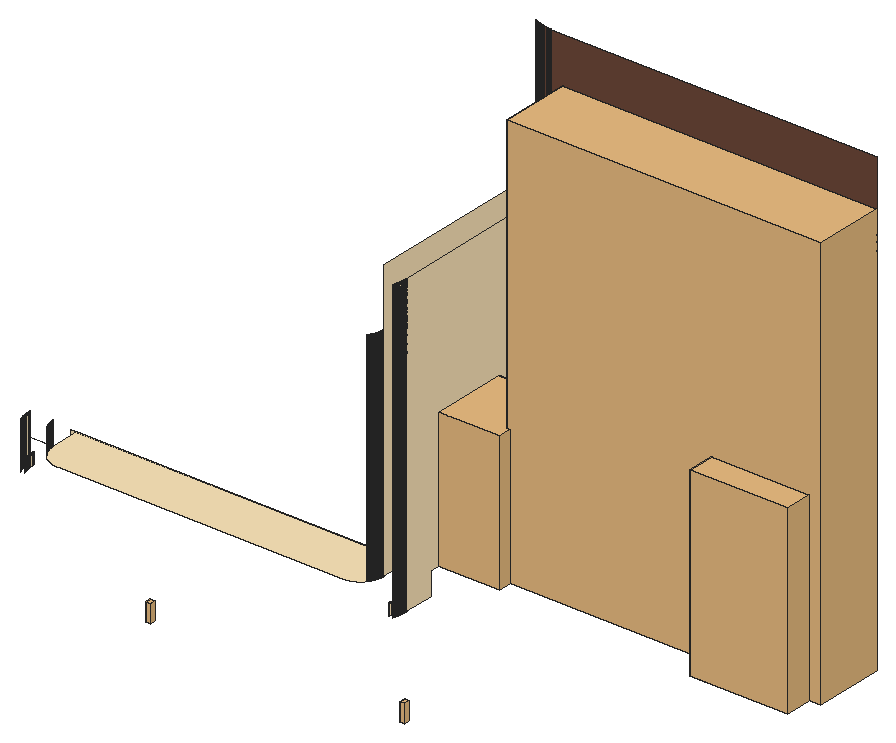
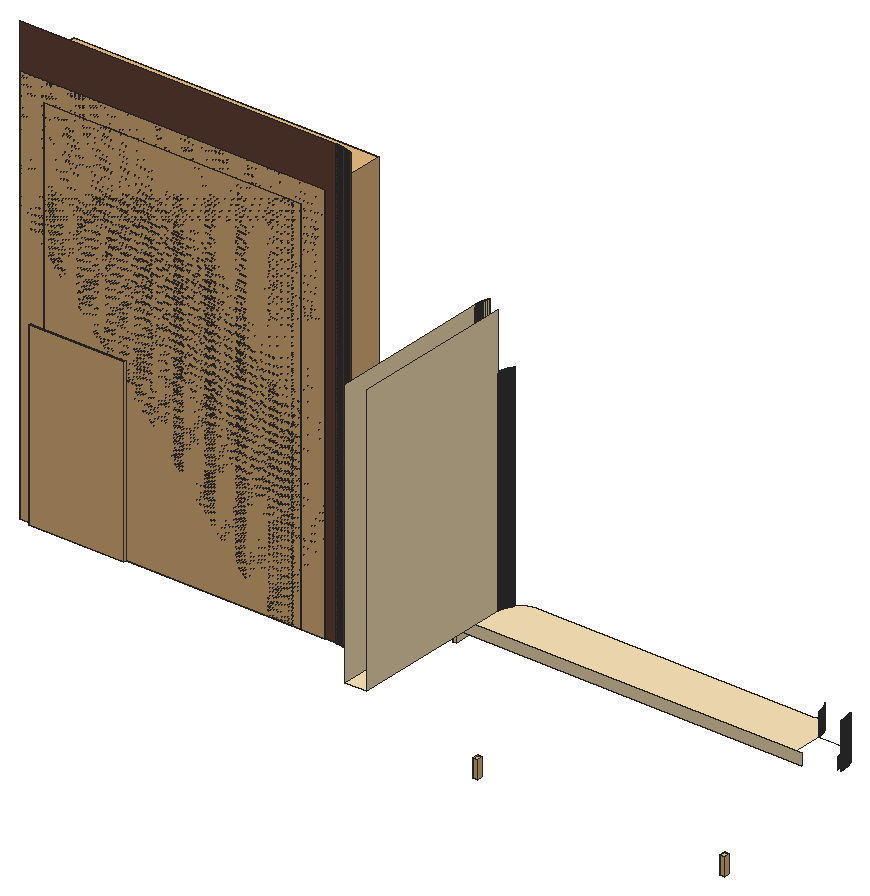
# SketchUp Ruby script. Lengths in inches.
U = 1.inch
M = Sketchup.active_model
def pt(a) = Geom::Point3d.new(a.map { |v| v * U })
def face(e, loops, mat)
  f = e.add_face(loops[0].map { |a| pt(a) })
  loops[1..].each { |l| e.add_face(l.map { |a| pt(a) }).erase! }
  f.material = f.back_material = mat if mat
  f
end
# faces: each face lists its corners as indices into pts; further lists are holes
def faces(e, pts, list, mat = nil) = list.each { |f| face(e, (f[0].is_a?(Array) ? f : [f]).map { |l| l.map { |i| pts[i] } }, mat) }
# xy, xz, yz: faces in a plane at the given z, y or x. An outline is a flat list of corners, or four numbers for a rectangle; further outlines are holes
def ring(l) = l.size == 4 ? [[l[0], l[1]], [l[2], l[1]], [l[2], l[3]], [l[0], l[3]]] : l.each_slice(2).to_a
def flat(e, list, mat, &to3) = list.each { |f| face(e, (f[0].is_a?(Array) ? f : [f]).map { |l| ring(l).map { |u, v| to3.(u, v) } }, mat) }
def xy(e, z, list, mat = nil) = flat(e, list, mat) { |x, y| [x, y, z] }
def xz(e, y, list, mat = nil) = flat(e, list, mat) { |x, z| [x, y, z] }
def yz(e, x, list, mat = nil) = flat(e, list, mat) { |y, z| [x, y, z] }
def lines(e, pts, list) = list.each { |a, b| e.add_line(pt(pts[a]), pt(pts[b])) }
# prism: a flat outline (further loops are holes) pulled along v
def prism(e, loops, v, mat = nil)
  f = face(e, loops, mat); d = Geom::Vector3d.new(v.map { |x| x * U })
  f.pushpull(f.normal.samedirection?(d) ? d.length : -d.length)
end
def box(e, o, s, mat = nil) = prism(e, [[o, [o[0] + s[0], o[1], o[2]], [o[0] + s[0], o[1] + s[1], o[2]], [o[0], o[1] + s[1], o[2]]]], [0, 0, s[2]], mat)
def at(x, y, z, deg = 0) = Geom::Transformation.translation(pt([x, y, z])) * Geom::Transformation.rotation(ORIGIN, Z_AXIS, deg.degrees)
def axes(o, x, y, z) = Geom::Transformation.new([*x, 0, *y, 0, *z, 0, *pt(o).to_a, 1])
def part(name) = M.definitions.add(name)
# library, detail: a bought-in or finely detailed component or shape, given as its bounding box
def library(name, o, s) = part(name).tap { |d| box(d.entities, o, s) }
def detail(e, o, s) = box(e.add_group.entities, o, s)
def put(e, d, t, mat = nil) = e.add_instance(d, t).tap { |i| i.material = mat if mat }
def group(e, t, mat = nil) = e.add_group.tap { |g| g.transformation = t; g.material = mat if mat }.entities
root = M.entities
M.materials.add("1026 AP 7946 SUNNY SIDE UP").color = [254, 231, 186]
M.materials.add("1916 AP K226 Macadamia Cream-N").color = [109, 72, 58]
M.materials.add("[Wood Cherry Original]").color = [152, 86, 42]
c1 = library("WALL LIGHT 69",[4.19,4.05,-9.3],[4.61,5.7,18.16])
c2 = library("Group\#76",[0,0,0],[126.13,128.06,238.18])
c3 = library("Plant Alocasia Zebrina",[379.59,151.79,0],[31.79,38.67,71.44])
c4 = library("Group\#4",[0,-36,0],[156,36,214])
c5 = library("Group\#36",[0,-0.25,0],[137.28,0.25,203])
xy(root,132,[[29.81,227,177.25,227,177.375,227.01,177.5,227.01,177.63,227.02,177.75,227.02,177.88,227.03,178,227.04,178.13,227.05,178.25,227.07,178.38,227.08,178.5,227.09,178.63,227.11,178.75,227.13,178.88,227.15,179,227.17,179.25,227.21,179.37,227.24,179.49,227.26,179.62,227.29,179.98,227.38,180.11,227.41,180.23,227.44,180.35,227.48,180.47,227.51,180.71,227.59,180.83,227.625,180.95,227.67,181.06,227.71,181.18,227.75,181.3,227.8,181.42,227.84,181.53,227.89,181.65,227.9375,181.77,227.99,181.88,228.04,182,228.09,182.11,228.14,182.22,228.2,182.34,228.25,182.56,228.37,182.67,228.42,182.78,228.48,182.89,228.55,183.11,228.67,183.22,228.74,183.32,228.8,183.43,228.87,183.54,228.9375,183.64,229,183.75,229.08,184.05,229.29,184.15,229.37,184.26,229.44,184.35,229.52,184.45,229.6,184.55,229.67,184.75,229.83,184.84,229.92,184.9375,230,185.03,230.08,185.12,230.17,185.21,230.25,185.31,230.34,185.4,230.43,185.49,230.51,185.57,230.6,185.66,230.69,185.75,230.79,185.83,230.88,185.92,230.97,186,231.0625,186.08,231.16,186.17,231.25,186.33,231.45,186.4,231.55,186.48,231.65,186.56,231.74,186.63,231.85,186.71,231.95,186.92,232.25,187,232.36,187.0625,232.46,187.13,232.57,187.2,232.68,187.26,232.78,187.33,232.89,187.45,233.11,187.52,233.22,187.58,233.33,187.63,233.44,187.75,233.66,187.8,233.78,187.86,233.89,187.91,234,187.96,234.12,188.01,234.23,188.0625,234.35,188.11,234.47,188.16,234.58,188.2,234.7,188.25,234.82,188.29,234.94,188.33,235.05,188.375,235.17,188.41,235.29,188.49,235.53,188.52,235.65,188.56,235.77,188.59,235.89,188.62,236.02,188.71,236.38,188.74,236.51,188.76,236.63,188.79,236.75,188.83,237,188.85,237.12,188.87,237.25,188.89,237.37,188.91,237.5,188.92,237.62,188.93,237.75,188.95,237.87,188.96,238,188.97,238.12,188.98,238.25,188.98,238.37,188.99,238.5,188.99,238.625,189,238.75,189,254,18,254,18,238.76,18.01,238.53,18.02,238.29,18.04,238.06,18.06,237.82,18.08,237.59,18.11,237.36,18.17,237.01,18.1875,236.89,18.23,236.66,18.25,236.54,18.3,236.3125,18.36,236.08,18.42,235.86,18.45,235.74,18.52,235.52,18.55,235.4,18.66,235.07,18.78,234.74,19.05,234.08,19.15,233.87,19.2,233.76,19.36,233.45,19.47,233.24,19.53,233.14,19.65,232.93,19.89,232.53,20.02,232.33,20.15,232.14,20.22,232.04,20.36,231.85,20.43,231.76,20.58,231.57,20.72,231.39,21.03,231.03,21.1875,230.85,21.35,230.68,21.68,230.35,21.85,230.1875,22.03,230.03,22.39,229.72,22.48,229.65,22.66,229.5,23.04,229.22,23.24,229.09,23.43,228.96,23.63,228.83,24.03,228.59,24.24,228.47,24.66,228.25,25.08,228.05,25.74,227.78,25.96,227.7,26.18,227.625,26.52,227.52,26.63,227.48,26.86,227.42,27.08,227.36,27.3125,227.3,27.54,227.25,27.77,227.21,28.01,227.17,28.36,227.11,28.59,227.08,28.82,227.06,29.06,227.04,29.29,227.02,29.53,227.01],[189,254,201,326]],"1026 AP 7946 SUNNY SIDE UP")
xz(root,254,[[199,120,199,126,15.03,126,15.03,132,201,132,201,120]],"1026 AP 7946 SUNNY SIDE UP")
xz(root,302,[[224.53,132,224.76,370],[224.76,132,224.85,370],[224.85,132,225,370],[225,132,243.24,132,243.24,298,243.55,302.75,244.46,307.42,245.96,311.93,248.03,316.21,250.63,320.2,253.73,323.8125,257.25,327,261.16,329.71,265.39,331.9,269.86,333.52,274.5,334.5625,279.24,335,347.52,335,351.97,334.21,356.29,332.9,360.42,331.0625,364.3,328.74,367.87,325.97,371.07,322.79,373.87,319.24,376.22,315.38,378.08,311.26,379.43,306.95,380.25,302.51,380.52,298,380.52,132,393,132,393,370,225,370],[[243.24,132,380.52,132,380.52,298,380.25,302.51,379.43,306.95,378.08,311.26,376.22,315.38,373.87,319.24,371.07,322.79,367.87,325.97,364.3,328.74,360.42,331.0625,356.29,332.9,351.97,334.21,347.52,335,279.24,335,274.5,334.5625,269.86,333.52,265.39,331.9,261.16,329.71,257.25,327,253.73,323.8125,250.63,320.2,248.03,316.21,245.96,311.93,244.46,307.42,243.55,302.75,243.24,298],[305.52,138,347.52,333.89]]],"1916 AP K226 Macadamia Cream-N")
yz(root,6,[[238.49,120,238.72,144],[238.72,120,238.96,144],[238.96,120,239,132],[238.96,132,239,144]],"1026 AP 7946 SUNNY SIDE UP")
yz(root,8,[[238.53,120,238.74,126],[238.74,120,238.96,126],[238.96,120,238.99,126]],"1026 AP 7946 SUNNY SIDE UP")
yz(root,18,[[238.76,132,239,144],[239,132,239.01,144],[239.01,132,239.06,144]],"1026 AP 7946 SUNNY SIDE UP")
yz(root,188.98,[[238.25,132,238.37,246]],"1026 AP 7946 SUNNY SIDE UP")
yz(root,188.99,[[238.5,132,238.625,246]],"1026 AP 7946 SUNNY SIDE UP")
yz(root,189,[[238.75,132,239,246],[239,132,326,276]],"1026 AP 7946 SUNNY SIDE UP")
yz(root,199,[[238.54,120,238.77,126],[238.77,120,239,126],[239,120,254,126]],"1026 AP 7946 SUNNY SIDE UP")
yz(root,200.99,[[238.25,120,238.5,274]],"1026 AP 7946 SUNNY SIDE UP")
yz(root,201,[[238.75,120,239,274],[239,120,254,120,254,132,326,132,326,274,239,274]],"1026 AP 7946 SUNNY SIDE UP")
p = [[7.26,231.33,120],[7.34,231.1,120],[7.34,231.1,144],[7.26,231.33,144],[197.62,231.33,120],[197.54,231.12,120],
  [197.54,231.12,126],[197.62,231.33,126],[199.75,231.34,120],[199.75,231.34,274],[199.67,231.11,274],[199.67,231.11,120],
  [9.45,231.15,120],[9.37,231.36,120],[9.37,231.36,126],[9.45,231.15,126],[7.19,231.55,120],[7.19,231.55,144],
  [197.7,231.55,120],[197.7,231.55,126],[199.83,231.58,120],[199.83,231.58,274],[9.3,231.56,120],[9.3,231.56,126],
  [7.11,231.77,120],[7.11,231.77,144],[197.78,231.76,120],[197.78,231.76,126],[9.22,231.76,120],[9.22,231.76,126],
  [199.9,231.82,120],[199.9,231.82,274],[7.04,232,120],[7.04,232,144],[9.15,231.97,120],[9.15,231.97,126],
  [197.85,231.98,120],[197.85,231.98,126],[199.98,232.0625,120],[199.98,232.0625,274],[6.98,232.22,120],[6.98,232.22,144],
  [9.09,232.17,120],[9.09,232.17,126],[197.92,232.2,120],[197.92,232.2,126],[200.05,232.3,120],[200.05,232.3,274],
  [6.91,232.45,120],[6.91,232.45,144],[9.02,232.375,120],[9.02,232.375,126],[197.99,232.42,120],[197.99,232.42,126],
  [200.12,232.55,120],[200.12,232.55,274],[8.96,232.58,120],[8.96,232.58,126],[198.0625,232.64,120],[198.0625,232.64,126],
  [6.85,232.68,120],[6.85,232.68,144],[200.18,232.79,120],[200.18,232.79,274],[8.89,232.79,120],[8.89,232.79,126],
  [198.125,232.86,120],[198.125,232.86,126],[6.79,232.9,120],[6.79,232.9,144],[8.83,233,120],[8.83,233,126],
  [200.25,233.03,120],[200.25,233.03,274],[6.73,233.13,120],[6.73,233.13,144],[198.19,233.08,120],[198.19,233.08,126],
  [8.78,233.2,120],[8.78,233.2,126],[200.31,233.28,120],[200.31,233.28,274],[6.67,233.36,120],[6.67,233.36,144],
  [198.25,233.31,120],[198.25,233.31,126],[8.72,233.41,120],[8.72,233.41,126],[198.31,233.53,120],[198.31,233.53,126],
  [200.37,233.52,120],[200.37,233.52,274],[6.62,233.59,120],[6.62,233.59,144],[8.67,233.62,120],[8.67,233.62,126],
  [198.36,233.75,120],[198.36,233.75,126],[200.42,233.76,120],[200.42,233.76,274],[6.57,233.82,120],[6.57,233.82,144],
  [8.62,233.83,120],[8.62,233.83,126],[6.52,234.05,120],[6.52,234.05,144],[8.57,234.04,120],[8.57,234.04,126],
  [198.42,233.98,120],[198.42,233.98,126],[200.48,234.01,120],[200.48,234.01,274],[6.47,234.28,120],[6.47,234.28,144],
  [8.52,234.25,120],[8.52,234.25,126],[198.47,234.2,120],[198.47,234.2,126],[200.53,234.26,120],[200.53,234.26,274],
  [198.52,234.43,120],[198.52,234.43,126],[6.42,234.51,120],[6.42,234.51,144],[8.47,234.46,120],[8.47,234.46,126],
  [200.57,234.5,120],[200.57,234.5,274],[198.57,234.65,120],[198.57,234.65,126],[6.38,234.74,120],[6.38,234.74,144],
  [8.43,234.67,120],[8.43,234.67,126],[200.62,234.75,120],[200.62,234.75,274],[6.34,234.97,120],[6.34,234.97,144],
  [8.39,234.88,120],[8.39,234.88,126],[198.61,234.88,120],[198.61,234.88,126],[200.66,235,120],[200.66,235,274],
  [8.35,235.1,120],[8.35,235.1,126],[198.65,235.1,120],[198.65,235.1,126],[6.3,235.21,120],[6.3,235.21,144],
  [200.7,235.25,120],[200.7,235.25,274],[8.3125,235.31,120],[8.3125,235.31,126],[198.69,235.33,120],[198.69,235.33,126],
  [6.27,235.4375,120],[6.27,235.4375,144],[200.74,235.49,120],[200.74,235.49,274],[8.28,235.52,120],[8.28,235.52,126],
  [198.73,235.56,120],[198.73,235.56,126],[6.23,235.67,120],[6.23,235.67,144],[8.24,235.74,120],[8.24,235.74,126],
  [200.78,235.74,120],[200.78,235.74,274],[198.76,235.79,120],[198.76,235.79,126],[6.2,235.9,120],[6.2,235.9,144],
  [8.21,235.95,120],[8.21,235.95,126],[200.8125,235.99,120],[200.8125,235.99,274],[198.8,236.01,120],[198.8,236.01,126],
  [6.17,236.14,120],[6.17,236.14,144],[8.18,236.16,120],[8.18,236.16,126],[198.83,236.24,120],[198.83,236.24,126],
  [200.84,236.24,120],[200.84,236.24,274],[6.14,236.37,120],[6.14,236.37,144],[8.16,236.375,120],[8.16,236.375,126],
  [198.85,236.47,120],[198.85,236.47,126],[200.87,236.49,120],[200.87,236.49,274],[6.12,236.61,120],[6.12,236.61,144],
  [8.13,236.59,120],[8.13,236.59,126],[198.88,236.7,120],[198.88,236.7,126],[200.89,236.74,120],[200.89,236.74,274],
  [6.1,236.84,120],[6.1,236.84,144],[8.11,236.81,120],[8.11,236.81,126],[198.9,236.93,120],[198.9,236.93,126],
  [200.92,236.99,120],[200.92,236.99,274],[6.08,237.08,120],[6.08,237.08,144],[8.09,237.02,120],[8.09,237.02,126],
  [198.92,237.16,120],[198.92,237.16,126],[8.07,237.24,120],[8.07,237.24,126],[200.9375,237.24,120],[200.9375,237.24,274],
  [6.06,237.31,120],[6.06,237.31,144],[8.05,237.45,120],[8.05,237.45,126],[198.94,237.39,120],[198.94,237.39,126],
  [200.95,237.49,120],[200.95,237.49,274],[6.04,237.54,120],[6.04,237.54,144],[198.96,237.62,120],[198.96,237.62,126],
  [6.03,237.78,120],[6.03,237.78,144],[8.04,237.67,120],[8.04,237.67,126],[200.97,237.74,120],[200.97,237.74,274],
  [198.97,237.85,120],[198.97,237.85,126],[8.03,237.88,120],[8.03,237.88,126],[200.98,237.99,120],[200.98,237.99,274],
  [6.02,238.01,120],[6.02,238.01,144],[198.98,238.08,120],[198.98,238.08,126],[8.02,238.1,120],[8.02,238.1,126],
  [6.01,238.25,120],[6.01,238.25,144],[200.99,238.25,120],[200.99,238.25,274],[8.01,238.3125,120],[8.01,238.3125,126],
  [198.99,238.31,120],[198.99,238.31,126],[6,238.49,120],[6,238.49,144],[8,238.53,120],[8,238.53,126],
  [199,238.54,120],[199,238.54,126],[201,238.75,120],[201,238.75,274],[200.99,238.5,274],[200.99,238.5,120],
  [20.875,231.21,132],[20.72,231.39,132],[20.72,231.39,144],[20.875,231.21,144],[186.17,231.25,132],[186.17,231.25,246],
  [186.25,231.35,246],[186.25,231.35,132],[20.58,231.57,132],[20.58,231.57,144],[186.33,231.45,246],[186.33,231.45,132],
  [186.4,231.55,246],[186.4,231.55,132],[186.48,231.65,246],[186.48,231.65,132],[20.43,231.76,132],[20.43,231.76,144],
  [186.56,231.74,246],[186.56,231.74,132],[186.63,231.85,246],[186.63,231.85,132],[20.36,231.85,132],[20.36,231.85,144],
  [186.71,231.95,246],[186.71,231.95,132],[20.22,232.04,132],[20.22,232.04,144],[186.78,232.05,246],[186.78,232.05,132],
  [20.15,232.14,132],[20.15,232.14,144],[186.85,232.15,246],[186.85,232.15,132],[20.02,232.33,132],[20.02,232.33,144],
  [186.92,232.25,246],[186.92,232.25,132],[19.89,232.53,132],[19.89,232.53,144],[187,232.36,246],[187,232.36,132],
  [187.0625,232.46,246],[187.0625,232.46,132],[19.83,232.63,132],[19.83,232.63,144],[187.13,232.57,246],[187.13,232.57,132],
  [19.71,232.83,132],[19.71,232.83,144],[187.2,232.68,246],[187.2,232.68,132],[187.26,232.78,246],[187.26,232.78,132],
  [19.65,232.93,132],[19.65,232.93,144],[187.33,232.89,246],[187.33,232.89,132],[19.53,233.14,132],[19.53,233.14,144],
  [187.39,233,246],[187.39,233,132],[187.45,233.11,246],[187.45,233.11,132],[19.47,233.24,132],[19.47,233.24,144],
  [187.52,233.22,246],[187.52,233.22,132],[19.36,233.45,132],[19.36,233.45,144],[187.58,233.33,246],[187.58,233.33,132],
  [187.63,233.44,246],[187.63,233.44,132],[19.2,233.76,132],[19.2,233.76,144],[187.69,233.55,246],[187.69,233.55,132],
  [187.75,233.66,246],[187.75,233.66,132],[187.8,233.78,246],[187.8,233.78,132],[19.15,233.87,132],[19.15,233.87,144],
  [187.86,233.89,246],[187.86,233.89,132],[19.05,234.08,132],[19.05,234.08,144],[187.91,234,246],[187.91,234,132],
  [187.96,234.12,246],[187.96,234.12,132],[18.96,234.3,132],[18.96,234.3,144],[188.01,234.23,246],[188.01,234.23,132],
  [188.0625,234.35,246],[188.0625,234.35,132],[18.87,234.52,132],[18.87,234.52,144],[188.11,234.47,246],[188.11,234.47,132],
  [18.78,234.74,132],[18.78,234.74,144],[188.16,234.58,246],[188.16,234.58,132],[188.2,234.7,246],[188.2,234.7,132],
  [18.74,234.85,132],[18.74,234.85,144],[188.25,234.82,246],[188.25,234.82,132],[18.66,235.07,132],[18.66,235.07,144],
  [188.29,234.94,246],[188.29,234.94,132],[188.33,235.05,246],[188.33,235.05,132],[18.55,235.4,132],[18.55,235.4,144],
  [188.375,235.17,246],[188.375,235.17,132],[188.41,235.29,246],[188.41,235.29,132],[188.45,235.41,246],[188.45,235.41,132],
  [18.52,235.52,132],[18.52,235.52,144],[188.49,235.53,246],[188.49,235.53,132],[18.45,235.74,132],[18.45,235.74,144],
  [188.52,235.65,246],[188.52,235.65,132],[18.42,235.86,132],[18.42,235.86,144],[188.56,235.77,246],[188.56,235.77,132],
  [188.59,235.89,246],[188.59,235.89,132],[18.36,236.08,132],[18.36,236.08,144],[188.62,236.02,246],[188.62,236.02,132],
  [188.65,236.14,246],[188.65,236.14,132],[18.3,236.3125,132],[18.3,236.3125,144],[188.68,236.26,246],[188.68,236.26,132],
  [18.25,236.54,132],[18.25,236.54,144],[188.71,236.38,246],[188.71,236.38,132],[188.74,236.51,246],[188.74,236.51,132],
  [18.23,236.66,132],[18.23,236.66,144],[188.76,236.63,246],[188.76,236.63,132],[188.79,236.75,246],[188.79,236.75,132],
  [18.1875,236.89,132],[18.1875,236.89,144],[188.81,236.875,246],[188.81,236.875,132],[18.17,237.01,132],[18.17,237.01,144],
  [188.83,237,246],[188.83,237,132],[18.11,237.36,132],[18.11,237.36,144],[188.85,237.12,246],[188.85,237.12,132],
  [188.87,237.25,246],[188.87,237.25,132],[188.89,237.37,246],[188.89,237.37,132],[18.08,237.59,132],[18.08,237.59,144],
  [188.91,237.5,246],[188.91,237.5,132],[188.92,237.62,246],[188.92,237.62,132],[18.06,237.82,132],[18.06,237.82,144],
  [188.93,237.75,246],[188.93,237.75,132],[188.95,237.87,246],[188.95,237.87,132],[18.04,238.06,132],[18.04,238.06,144],
  [188.96,238,246],[188.96,238,132],[188.97,238.12,246],[188.97,238.12,132],[18.02,238.29,132],[18.02,238.29,144],
  [188.98,238.25,246],[188.98,238.25,132],[18.01,238.53,132],[18.01,238.53,144],[188.98,238.37,132],[188.98,238.37,246],
  [188.99,238.5,246],[188.99,238.5,132],[18,238.76,132],[18,238.76,144],[188.99,238.625,132],[188.99,238.625,246],
  [189,238.75,246],[189,238.75,132],[223.59,302.04,132],[223.59,302.04,370],[223.35,302.06,370],[223.35,302.06,132],
  [223.82,302.03,132],[223.82,302.03,370],[224.06,302.02,132],[224.06,302.02,370],[224.29,302.01,132],[224.29,302.01,370],
  [224.53,302,132],[224.53,302,370],[222.41,302.14,132],[222.41,302.14,370],[222.18,302.17,370],[222.18,302.17,132],
  [222.65,302.12,132],[222.65,302.12,370],[222.88,302.09,132],[222.88,302.09,370],[223.12,302.07,132],[223.12,302.07,370],
  [221.71,302.23,132],[221.71,302.23,370],[221.48,302.26,370],[221.48,302.26,132],[221.95,302.2,132],[221.95,302.2,370],
  [221.01,302.33,132],[221.01,302.33,370],[220.78,302.375,370],[220.78,302.375,132],[221.25,302.3,132],[221.25,302.3,370],
  [220.55,302.42,132],[220.55,302.42,370],[220.32,302.46,370],[220.32,302.46,132],[220.09,302.51,132],[220.09,302.51,370],
  [219.86,302.56,370],[219.86,302.56,132],[219.625,302.61,132],[219.625,302.61,370],[219.4,302.66,370],[219.4,302.66,132],
  [219.17,302.72,132],[219.17,302.72,370],[218.94,302.78,370],[218.94,302.78,132],[218.71,302.84,132],[218.71,302.84,370],
  [218.49,302.9,370],[218.49,302.9,132],[218.26,302.97,370],[218.26,302.97,132],[218.03,303.03,132],[218.03,303.03,370],
  [217.81,303.1,370],[217.81,303.1,132],[217.58,303.17,370],[217.58,303.17,132],[217.36,303.25,132],[217.36,303.25,370],
  [217.14,303.32,370],[217.14,303.32,132],[216.91,303.4,370],[216.91,303.4,132],[216.69,303.48,370],[216.69,303.48,132],
  [216.47,303.57,370],[216.47,303.57,132],[216.25,303.65,370],[216.25,303.65,132],[216.03,303.74,132],[216.03,303.74,370],
  [215.82,303.83,370],[215.82,303.83,132],[215.6,303.92,370],[215.6,303.92,132],[215.38,304.01,370],[215.38,304.01,132],
  [215.17,304.11,370],[215.17,304.11,132],[18,239.06,132],[6,239,132]]
faces(root,p,[[0,1,2,3],[4,5,6,7],[8,9,10,11],[12,13,14,15],[16,0,3,17],[18,4,7,19],[20,21,9,8],[13,22,23,14],
  [24,16,17,25],[26,18,19,27],[22,28,29,23],[30,31,21,20],[32,24,25,33],[28,34,35,29],[36,26,27,37],[38,39,31,30],
  [40,32,33,41],[34,42,43,35],[44,36,37,45],[46,47,39,38],[48,40,41,49],[42,50,51,43],[52,44,45,53],[54,55,47,46],
  [50,56,57,51],[58,52,53,59],[60,48,49,61],[62,63,55,54],[56,64,65,57],[66,58,59,67],[68,60,61,69],[64,70,71,65],
  [72,73,63,62],[74,68,69,75],[76,66,67,77],[70,78,79,71],[80,81,73,72],[82,74,75,83],[84,76,77,85],[78,86,87,79],
  [88,84,85,89],[90,91,81,80],[92,82,83,93],[86,94,95,87],[96,88,89,97],[98,99,91,90],[100,92,93,101],[94,102,103,95],
  [104,100,101,105],[102,106,107,103],[108,96,97,109],[110,111,99,98],[112,104,105,113],[106,114,115,107],[116,108,109,117],[118,119,111,110],
  [120,116,117,121],[122,112,113,123],[114,124,125,115],[126,127,119,118],[128,120,121,129],[130,122,123,131],[124,132,133,125],[134,135,127,126],
  [136,130,131,137],[132,138,139,133],[140,128,129,141],[142,143,135,134],[138,144,145,139],[146,140,141,147],[148,136,137,149],[150,151,143,142],
  [144,152,153,145],[154,146,147,155],[156,148,149,157],[158,159,151,150],[152,160,161,153],[162,154,155,163],[164,156,157,165],[160,166,167,161],
  [168,169,159,158],[170,162,163,171],[172,164,165,173],[166,174,175,167],[176,177,169,168],[178,170,171,179],[180,172,173,181],[174,182,183,175],
  [184,178,179,185],[186,187,177,176],[188,180,181,189],[182,190,191,183],[192,184,185,193],[194,195,187,186],[196,188,189,197],[190,198,199,191],
  [200,192,193,201],[202,203,195,194],[204,196,197,205],[198,206,207,199],[208,200,201,209],[210,211,203,202],[212,204,205,213],[206,214,215,207],
  [216,208,209,217],[214,218,219,215],[220,221,211,210],[222,212,213,223],[218,224,225,219],[226,216,217,227],[228,229,221,220],[230,222,223,231],
  [232,226,227,233],[234,230,231,235],[224,236,237,225],[238,239,229,228],[240,232,233,241],[236,242,243,237],[244,245,239,238],[246,234,235,247],
  [248,240,241,249],[242,250,251,243],[252,246,247,253],[254,255,245,244],[250,256,257,251],[258,248,249,259],[260,252,253,261],[256,262,263,257],
  [264,258,259,265],[266,267,268,269],[270,271,272,273],[274,275,276,277],[271,278,279,272],[277,276,280,281],[281,280,282,283],[283,282,284,285],
  [278,286,287,279],[285,284,288,289],[289,288,290,291],[286,292,293,287],[291,290,294,295],[292,296,297,293],[295,294,298,299],[296,300,301,297],
  [299,298,302,303],[300,304,305,301],[303,302,306,307],[304,308,309,305],[307,306,310,311],[311,310,312,313],[308,314,315,309],[313,312,316,317],
  [314,318,319,315],[317,316,320,321],[321,320,322,323],[318,324,325,319],[323,322,326,327],[324,328,329,325],[327,326,330,331],[331,330,332,333],
  [328,334,335,329],[333,332,336,337],[334,338,339,335],[337,336,340,341],[341,340,342,343],[338,344,345,339],[343,342,346,347],[347,346,348,349],
  [349,348,350,351],[344,352,353,345],[351,350,354,355],[352,356,357,353],[355,354,358,359],[359,358,360,361],[356,362,363,357],[361,360,364,365],
  [365,364,366,367],[362,368,369,363],[367,366,370,371],[368,372,373,369],[371,370,374,375],[375,374,376,377],[372,378,379,373],[377,376,380,381],
  [378,382,383,379],[381,380,384,385],[385,384,386,387],[382,388,389,383],[387,386,390,391],[391,390,392,393],[393,392,394,395],[388,396,397,389],
  [395,394,398,399],[396,400,401,397],[399,398,402,403],[400,404,405,401],[403,402,406,407],[407,406,408,409],[404,410,411,405],[409,408,412,413],
  [413,412,414,415],[410,416,417,411],[415,414,418,419],[416,420,421,417],[419,418,422,423],[423,422,424,425],[420,426,427,421],[425,424,428,429],
  [429,428,430,431],[426,432,433,427],[431,430,434,435],[432,436,437,433],[435,434,438,439],[436,440,441,437],[439,438,442,443],[443,442,444,445],
  [445,444,446,447],[440,448,449,441],[447,446,450,451],[451,450,452,453],[448,454,455,449],[453,452,456,457],[457,456,458,459],[454,460,461,455],
  [459,458,462,463],[463,462,464,465],[460,466,467,461],[465,464,468,469],[466,470,471,467],[472,473,474,475],[470,476,477,471],[478,479,480,481]],"1026 AP 7946 SUNNY SIDE UP")
faces(root,p,[[482,483,484,485],[486,487,483,482],[488,489,487,486],[490,491,489,488],[492,493,491,490],[494,495,496,497],[498,499,495,494],[500,501,499,498],
  [502,503,501,500],[485,484,503,502],[504,505,506,507],[508,509,505,504],[497,496,509,508],[510,511,512,513],[514,515,511,510],[507,506,515,514],
  [516,517,518,519],[513,512,517,516],[520,521,522,523],[519,518,521,520],[524,525,526,527],[523,522,525,524],[528,529,530,531],[527,526,529,528],
  [532,533,534,535],[531,530,533,532],[535,534,536,537],[538,539,540,541],[537,536,539,538],[541,540,542,543],[544,545,546,547],[543,542,545,544],
  [547,546,548,549],[549,548,550,551],[551,550,552,553],[553,552,554,555],[556,557,558,559],[555,554,557,556],[559,558,560,561],[561,560,562,563],
  [563,562,564,565]],"1916 AP K226 Macadamia Cream-N")
lines(root,p,[[566,567]])
put(root,c1,axes([185.45,248.93,63.55],[0.52,0,0],[0,0.52,0],[0,0,0.52]))
put(root,c1,axes([54.01,248.93,63.55],[0.52,0,0],[0,0.52,0],[0,0,0.52]))
put(root,c2,axes([336.6875,252.07,131.98],[0.4,0,0],[0,0.4,0],[0,0,0.4]),"1026 AP 7946 SUNNY SIDE UP")
put(root,c3,at(-178.75,107.24,132),"1026 AP 7946 SUNNY SIDE UP")
put(root,c4,axes([230.76,302,132],[1.04,0,0],[0,1,0],[0,0,1]),"1026 AP 7946 SUNNY SIDE UP")
put(root,c5,at(243.24,302,132),"[Wood Cherry Original]")
